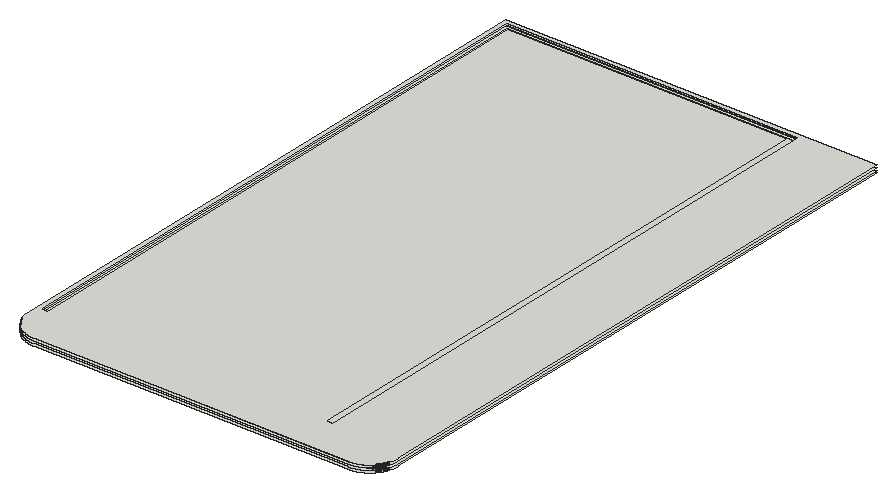
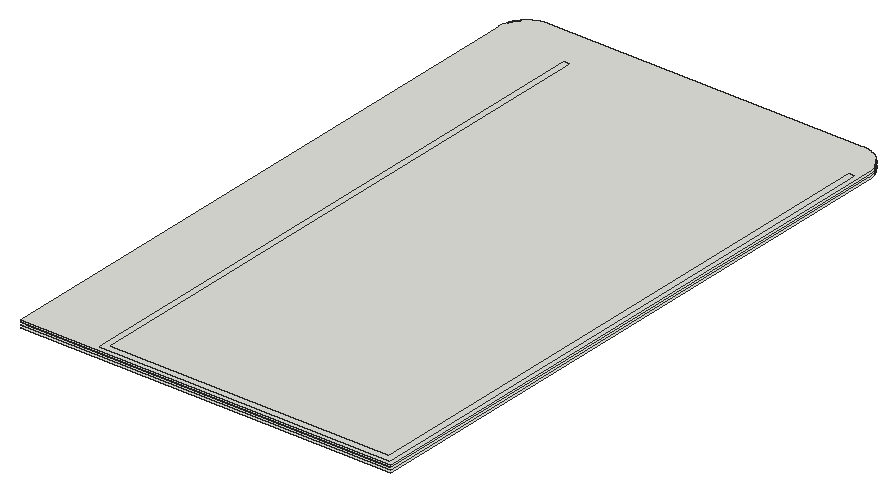
# SketchUp Ruby script. Lengths in inches.
U = 1.inch
M = Sketchup.active_model
def pt(a) = Geom::Point3d.new(a.map { |v| v * U })
def face(e, loops, mat)
  f = e.add_face(loops[0].map { |a| pt(a) })
  loops[1..].each { |l| e.add_face(l.map { |a| pt(a) }).erase! }
  f.material = f.back_material = mat if mat
  f
end
# faces: each face lists its corners as indices into pts; further lists are holes
def faces(e, pts, list, mat = nil) = list.each { |f| face(e, (f[0].is_a?(Array) ? f : [f]).map { |l| l.map { |i| pts[i] } }, mat) }
# xy, xz, yz: faces in a plane at the given z, y or x. An outline is a flat list of corners, or four numbers for a rectangle; further outlines are holes
def ring(l) = l.size == 4 ? [[l[0], l[1]], [l[2], l[1]], [l[2], l[3]], [l[0], l[3]]] : l.each_slice(2).to_a
def flat(e, list, mat, &to3) = list.each { |f| face(e, (f[0].is_a?(Array) ? f : [f]).map { |l| ring(l).map { |u, v| to3.(u, v) } }, mat) }
def xy(e, z, list, mat = nil) = flat(e, list, mat) { |x, y| [x, y, z] }
def xz(e, y, list, mat = nil) = flat(e, list, mat) { |x, z| [x, y, z] }
def yz(e, x, list, mat = nil) = flat(e, list, mat) { |y, z| [x, y, z] }
def lines(e, pts, list) = list.each { |a, b| e.add_line(pt(pts[a]), pt(pts[b])) }
# prism: a flat outline (further loops are holes) pulled along v
def prism(e, loops, v, mat = nil)
  f = face(e, loops, mat); d = Geom::Vector3d.new(v.map { |x| x * U })
  f.pushpull(f.normal.samedirection?(d) ? d.length : -d.length)
end
def box(e, o, s, mat = nil) = prism(e, [[o, [o[0] + s[0], o[1], o[2]], [o[0] + s[0], o[1] + s[1], o[2]], [o[0], o[1] + s[1], o[2]]]], [0, 0, s[2]], mat)
def at(x, y, z, deg = 0) = Geom::Transformation.translation(pt([x, y, z])) * Geom::Transformation.rotation(ORIGIN, Z_AXIS, deg.degrees)
def axes(o, x, y, z) = Geom::Transformation.new([*x, 0, *y, 0, *z, 0, *pt(o).to_a, 1])
def part(name) = M.definitions.add(name)
# library, detail: a bought-in or finely detailed component or shape, given as its bounding box
def library(name, o, s) = part(name).tap { |d| box(d.entities, o, s) }
def detail(e, o, s) = box(e.add_group.entities, o, s)
def put(e, d, t, mat = nil) = e.add_instance(d, t).tap { |i| i.material = mat if mat }
def group(e, t, mat = nil) = e.add_group.tap { |g| g.transformation = t; g.material = mat if mat }.entities
root = M.entities
xy(root,392.81,[[25.72,144,25.41,144.01,25.09,144.02,24.78,144.03,24.46,144.05,24.15,144.07,23.84,144.1,23.52,144.13,23.21,144.17,22.9,144.2,22.59,144.25,22.27,144.29,21.96,144.35,21.65,144.4,21.35,144.46,21.04,144.52,20.42,144.66,20.12,144.74,19.8125,144.82,19.51,144.9,18.61,145.17,18.31,145.27,18.01,145.375,17.72,145.48,17.42,145.59,16.26,146.07,15.97,146.2,15.6875,146.34,15.4,146.47,15.125,146.61,14.84,146.76,14.57,146.91,14.29,147.06,14.02,147.21,13.75,147.37,13.48,147.54,13.21,147.7,12.94,147.87,12.68,148.04,12.16,148.4,11.91,148.58,11.65,148.77,11.4,148.96,11.16,149.15,10.91,149.35,10.43,149.75,10.1875,149.95,9.95,150.16,9.49,150.59,9.26,150.81,8.82,151.25,8.6,151.48,8.39,151.71,8.17,151.94,7.96,152.17,7.56,152.65,7.36,152.9,7.16,153.14,6.59,153.89,6.41,154.15,6.23,154.4,6.05,154.67,5.71,155.19,5.54,155.46,5.06,156.27,4.91,156.55,4.76,156.82,4.48,157.38,4.34,157.67,4.21,157.95,4.08,158.24,3.95,158.52,3.83,158.8125,3.71,159.11,3.49,159.69,3.38,159.99,3.28,160.28,3.08,160.88,2.9,161.48,2.82,161.79,2.74,162.09,2.66,162.4,2.59,162.7,2.53,163.01,2.46,163.32,2.4,163.625,2.35,163.93,2.25,164.55,2.21,164.87,2.13,165.49,2.1,165.8,2.07,166.12,2.03,166.74,2.02,167.06,2,167.68,2,672,314.45,672,314.45,167.37,314.43,167.06,314.42,166.74,314.38,166.12,314.35,165.8,314.29,165.18,314.25,164.87,314.2,164.55,314.16,164.24,314.11,163.93,313.99,163.32,313.93,163.01,313.86,162.7,313.79,162.4,313.71,162.09,313.63,161.79,313.55,161.48,313.28,160.58,313.18,160.28,313.07,159.99,312.97,159.69,312.86,159.4,312.74,159.11,312.625,158.8125,312.5,158.52,312.375,158.24,312.25,157.95,312.11,157.67,311.97,157.38,311.83,157.1,311.6875,156.82,311.54,156.55,311.39,156.27,310.75,155.19,310.58,154.93,310.4,154.67,310.23,154.4,310.05,154.15,309.86,153.89,309.68,153.64,309.49,153.39,309.29,153.14,309.1,152.9,308.9,152.65,308.69,152.41,308.49,152.17,308.07,151.71,307.63,151.25,307.19,150.81,306.96,150.59,306.5,150.16,306.27,149.95,305.79,149.55,305.54,149.35,305.3,149.15,304.55,148.58,303.77,148.04,303.51,147.87,303.24,147.7,302.98,147.54,302.71,147.37,302.4375,147.21,302.16,147.06,301.89,146.91,301.33,146.61,301.05,146.47,300.77,146.34,300.48,146.2,300.19,146.07,299.91,145.95,299.62,145.83,299.32,145.71,299.03,145.59,298.74,145.48,298.14,145.27,297.85,145.17,297.55,145.08,297.24,144.99,296.94,144.9,296.64,144.82,296.33,144.74,296.03,144.66,295.72,144.59,295.42,144.52,294.8,144.4,294.49,144.35,294.18,144.29,293.87,144.25,293.56,144.2,293.24,144.17,292.93,144.13,292.62,144.1,292.3,144.07,291.68,144.03,291.36,144.02,291.05,144.01,290.73,144]])
xy(root,394.81,[[[25.72,144,290.73,144,291.05,144.01,291.36,144.02,291.68,144.03,292.3,144.07,292.62,144.1,292.93,144.13,293.24,144.17,293.56,144.2,293.87,144.25,294.18,144.29,294.49,144.35,294.8,144.4,295.42,144.52,295.72,144.59,296.03,144.66,296.33,144.74,296.64,144.82,296.94,144.9,297.24,144.99,297.55,145.08,297.85,145.17,298.14,145.27,298.74,145.48,299.03,145.59,299.32,145.71,299.62,145.83,299.91,145.95,300.19,146.07,300.48,146.2,300.77,146.34,301.05,146.47,301.33,146.61,301.89,146.91,302.16,147.06,302.4375,147.21,302.71,147.37,302.98,147.54,303.24,147.7,303.51,147.87,303.77,148.04,304.55,148.58,305.3,149.15,305.54,149.35,305.79,149.55,306.27,149.95,306.5,150.16,306.96,150.59,307.19,150.81,307.63,151.25,308.07,151.71,308.49,152.17,308.69,152.41,308.9,152.65,309.1,152.9,309.29,153.14,309.49,153.39,309.68,153.64,309.86,153.89,310.05,154.15,310.23,154.4,310.4,154.67,310.58,154.93,310.75,155.19,311.39,156.27,311.54,156.55,311.6875,156.82,311.83,157.1,311.97,157.38,312.11,157.67,312.25,157.95,312.375,158.24,312.5,158.52,312.625,158.8125,312.74,159.11,312.86,159.4,312.97,159.69,313.07,159.99,313.18,160.28,313.28,160.58,313.55,161.48,313.63,161.79,313.71,162.09,313.79,162.4,313.86,162.7,313.93,163.01,313.99,163.32,314.11,163.93,314.16,164.24,314.2,164.55,314.25,164.87,314.29,165.18,314.35,165.8,314.38,166.12,314.42,166.74,314.43,167.06,314.45,167.37,314.45,672,2,672,2,167.68,2.02,167.06,2.03,166.74,2.07,166.12,2.1,165.8,2.13,165.49,2.21,164.87,2.25,164.55,2.35,163.93,2.4,163.625,2.46,163.32,2.53,163.01,2.59,162.7,2.66,162.4,2.74,162.09,2.82,161.79,2.9,161.48,3.08,160.88,3.28,160.28,3.38,159.99,3.49,159.69,3.71,159.11,3.83,158.8125,3.95,158.52,4.08,158.24,4.21,157.95,4.34,157.67,4.48,157.38,4.76,156.82,4.91,156.55,5.06,156.27,5.54,155.46,5.71,155.19,6.05,154.67,6.23,154.4,6.41,154.15,6.59,153.89,7.16,153.14,7.36,152.9,7.56,152.65,7.96,152.17,8.17,151.94,8.39,151.71,8.6,151.48,8.82,151.25,9.26,150.81,9.49,150.59,9.95,150.16,10.1875,149.95,10.43,149.75,10.91,149.35,11.16,149.15,11.4,148.96,11.65,148.77,11.91,148.58,12.16,148.4,12.68,148.04,12.94,147.87,13.21,147.7,13.48,147.54,13.75,147.37,14.02,147.21,14.29,147.06,14.57,146.91,14.84,146.76,15.125,146.61,15.4,146.47,15.6875,146.34,15.97,146.2,16.26,146.07,17.42,145.59,17.72,145.48,18.01,145.375,18.31,145.27,18.61,145.17,19.51,144.9,19.8125,144.82,20.12,144.74,20.42,144.66,21.04,144.52,21.35,144.46,21.65,144.4,21.96,144.35,22.27,144.29,22.59,144.25,22.9,144.2,23.21,144.17,23.52,144.13,23.84,144.1,24.15,144.07,24.46,144.05,24.78,144.03,25.09,144.02,25.41,144.01],[25.75,146,24.88,146.03,24.59,146.05,24.31,146.07,24.02,146.09,23.44,146.15,23.16,146.1875,22.87,146.23,22.59,146.27,22.3,146.32,21.74,146.42,21.45,146.48,21.17,146.54,20.05,146.82,19.78,146.9,19.22,147.08,18.68,147.26,18.14,147.46,17.87,147.57,17.6,147.67,17.34,147.79,17.07,147.9,16.55,148.14,15.77,148.53,15.52,148.67,15.27,148.8,15.02,148.95,14.77,149.09,14.52,149.24,14.28,149.39,14.03,149.55,13.55,149.87,13.32,150.03,13.08,150.2,12.85,150.37,12.62,150.55,12.39,150.72,12.17,150.9,11.94,151.09,11.72,151.27,11.51,151.46,11.29,151.65,11.08,151.84,10.45,152.44,9.85,153.07,9.47,153.49,9.09,153.93,8.91,154.15,8.55,154.61,8.04,155.3,7.71,155.78,7.55,156.02,7.25,156.5,6.95,157,6.67,157.5,6.53,157.76,6.4,158.01,6.27,158.27,6.15,158.53,6.02,158.79,5.9,159.05,5.79,159.32,5.68,159.58,5.46,160.12,5.26,160.66,5.08,161.2,4.99,161.48,4.91,161.75,4.75,162.31,4.68,162.58,4.54,163.14,4.48,163.43,4.42,163.71,4.32,164.27,4.27,164.56,4.23,164.84,4.1875,165.13,4.15,165.41,4.09,165.99,4.07,166.27,4.03,166.85,4.02,167.14,4.01,167.42,4,167.71,4,670,312.45,670,312.45,167.42,312.4375,167.14,312.42,166.85,312.41,166.56,312.39,166.27,312.36,165.99,312.3,165.41,312.26,165.13,312.23,164.84,312.18,164.56,312.14,164.27,312.08,163.99,312.03,163.71,311.97,163.43,311.91,163.14,311.84,162.86,311.78,162.58,311.7,162.31,311.55,161.75,311.46,161.48,311.375,161.2,311.28,160.93,311.19,160.66,310.89,159.85,310.78,159.58,310.66,159.32,310.55,159.05,310.31,158.53,310.05,158.01,309.92,157.76,309.78,157.5,309.36,156.75,309.21,156.5,309.05,156.26,308.9,156.02,308.58,155.54,308.41,155.3,308.25,155.07,308.07,154.84,307.9,154.61,307.54,154.15,307.36,153.93,307.17,153.71,306.99,153.49,306.79,153.28,306.6,153.07,306,152.44,305.8,152.24,305.59,152.04,305.375,151.84,305.16,151.65,304.95,151.46,304.73,151.27,304.51,151.09,304.29,150.9,304.0625,150.72,303.83,150.55,303.6,150.37,303.14,150.03,302.18,149.39,301.93,149.24,301.6875,149.09,301.4375,148.95,301.1875,148.8,300.93,148.67,300.68,148.53,300.42,148.4,300.17,148.27,299.91,148.14,299.64,148.02,299.38,147.9,299.12,147.79,298.85,147.67,298.58,147.57,298.32,147.46,298.05,147.36,297.77,147.26,297.23,147.08,296.95,146.99,296.68,146.9,296.4,146.82,295.84,146.68,295.5625,146.61,295.28,146.54,294.72,146.42,294.43,146.37,293.87,146.27,293.58,146.23,293.3,146.1875,293.01,146.15,292.72,146.12,292.44,146.09,291.57,146.03,291.28,146.02,291,146.01,290.71,146]]])
xy(root,396.81,[[[25.72,144,25.41,144.01,25.09,144.02,24.78,144.03,24.46,144.05,24.15,144.07,23.84,144.1,23.52,144.13,23.21,144.17,22.9,144.2,22.59,144.25,22.27,144.29,21.96,144.35,21.65,144.4,21.35,144.46,21.04,144.52,20.42,144.66,20.12,144.74,19.8125,144.82,19.51,144.9,18.61,145.17,18.31,145.27,18.01,145.375,17.72,145.48,17.42,145.59,16.26,146.07,15.97,146.2,15.6875,146.34,15.4,146.47,15.125,146.61,14.84,146.76,14.57,146.91,14.29,147.06,14.02,147.21,13.75,147.37,13.48,147.54,13.21,147.7,12.94,147.87,12.68,148.04,12.16,148.4,11.91,148.58,11.65,148.77,11.4,148.96,11.16,149.15,10.91,149.35,10.43,149.75,10.1875,149.95,9.95,150.16,9.49,150.59,9.26,150.81,8.82,151.25,8.6,151.48,8.39,151.71,8.17,151.94,7.96,152.17,7.56,152.65,7.36,152.9,7.16,153.14,6.59,153.89,6.41,154.15,6.23,154.4,6.05,154.67,5.71,155.19,5.54,155.46,5.06,156.27,4.91,156.55,4.76,156.82,4.48,157.38,4.34,157.67,4.21,157.95,4.08,158.24,3.95,158.52,3.83,158.8125,3.71,159.11,3.49,159.69,3.38,159.99,3.28,160.28,3.08,160.88,2.9,161.48,2.82,161.79,2.74,162.09,2.66,162.4,2.59,162.7,2.53,163.01,2.46,163.32,2.4,163.625,2.35,163.93,2.25,164.55,2.21,164.87,2.13,165.49,2.1,165.8,2.07,166.12,2.03,166.74,2.02,167.06,2,167.68,2,672,314.45,672,314.45,167.37,314.43,167.06,314.42,166.74,314.38,166.12,314.35,165.8,314.29,165.18,314.25,164.87,314.2,164.55,314.16,164.24,314.11,163.93,313.99,163.32,313.93,163.01,313.86,162.7,313.79,162.4,313.71,162.09,313.63,161.79,313.55,161.48,313.28,160.58,313.18,160.28,313.07,159.99,312.97,159.69,312.86,159.4,312.74,159.11,312.625,158.8125,312.5,158.52,312.375,158.24,312.25,157.95,312.11,157.67,311.97,157.38,311.83,157.1,311.6875,156.82,311.54,156.55,311.39,156.27,310.75,155.19,310.58,154.93,310.4,154.67,310.23,154.4,310.05,154.15,309.86,153.89,309.68,153.64,309.49,153.39,309.29,153.14,309.1,152.9,308.9,152.65,308.69,152.41,308.49,152.17,308.07,151.71,307.63,151.25,307.19,150.81,306.96,150.59,306.5,150.16,306.27,149.95,305.79,149.55,305.54,149.35,305.3,149.15,304.55,148.58,303.77,148.04,303.51,147.87,303.24,147.7,302.98,147.54,302.71,147.37,302.4375,147.21,302.16,147.06,301.89,146.91,301.33,146.61,301.05,146.47,300.77,146.34,300.48,146.2,300.19,146.07,299.91,145.95,299.62,145.83,299.32,145.71,299.03,145.59,298.74,145.48,298.14,145.27,297.85,145.17,297.55,145.08,297.24,144.99,296.94,144.9,296.64,144.82,296.33,144.74,296.03,144.66,295.72,144.59,295.42,144.52,294.8,144.4,294.49,144.35,294.18,144.29,293.87,144.25,293.56,144.2,293.24,144.17,292.93,144.13,292.62,144.1,292.3,144.07,291.68,144.03,291.36,144.02,291.05,144.01,290.73,144],[25.75,146,290.71,146,291,146.01,291.28,146.02,291.57,146.03,292.44,146.09,292.72,146.12,293.01,146.15,293.3,146.1875,293.58,146.23,293.87,146.27,294.43,146.37,294.72,146.42,295.28,146.54,295.5625,146.61,295.84,146.68,296.4,146.82,296.68,146.9,296.95,146.99,297.23,147.08,297.77,147.26,298.05,147.36,298.32,147.46,298.58,147.57,298.85,147.67,299.12,147.79,299.38,147.9,299.64,148.02,299.91,148.14,300.17,148.27,300.42,148.4,300.68,148.53,300.93,148.67,301.1875,148.8,301.4375,148.95,301.6875,149.09,301.93,149.24,302.18,149.39,303.14,150.03,303.6,150.37,303.83,150.55,304.0625,150.72,304.29,150.9,304.51,151.09,304.73,151.27,304.95,151.46,305.16,151.65,305.375,151.84,305.59,152.04,305.8,152.24,306,152.44,306.6,153.07,306.79,153.28,306.99,153.49,307.17,153.71,307.36,153.93,307.54,154.15,307.9,154.61,308.07,154.84,308.25,155.07,308.41,155.3,308.58,155.54,308.9,156.02,309.05,156.26,309.21,156.5,309.36,156.75,309.78,157.5,309.92,157.76,310.05,158.01,310.31,158.53,310.55,159.05,310.66,159.32,310.78,159.58,310.89,159.85,311.19,160.66,311.28,160.93,311.375,161.2,311.46,161.48,311.55,161.75,311.7,162.31,311.78,162.58,311.84,162.86,311.91,163.14,311.97,163.43,312.03,163.71,312.08,163.99,312.14,164.27,312.18,164.56,312.23,164.84,312.26,165.13,312.3,165.41,312.36,165.99,312.39,166.27,312.41,166.56,312.42,166.85,312.4375,167.14,312.45,167.42,312.45,670,4,670,4,167.71,4.01,167.42,4.02,167.14,4.03,166.85,4.07,166.27,4.09,165.99,4.15,165.41,4.1875,165.13,4.23,164.84,4.27,164.56,4.32,164.27,4.42,163.71,4.48,163.43,4.54,163.14,4.68,162.58,4.75,162.31,4.91,161.75,4.99,161.48,5.08,161.2,5.26,160.66,5.46,160.12,5.68,159.58,5.79,159.32,5.9,159.05,6.02,158.79,6.15,158.53,6.27,158.27,6.4,158.01,6.53,157.76,6.67,157.5,6.95,157,7.25,156.5,7.55,156.02,7.71,155.78,8.04,155.3,8.55,154.61,8.91,154.15,9.09,153.93,9.47,153.49,9.85,153.07,10.45,152.44,11.08,151.84,11.29,151.65,11.51,151.46,11.72,151.27,11.94,151.09,12.17,150.9,12.39,150.72,12.62,150.55,12.85,150.37,13.08,150.2,13.32,150.03,13.55,149.87,14.03,149.55,14.28,149.39,14.52,149.24,14.77,149.09,15.02,148.95,15.27,148.8,15.52,148.67,15.77,148.53,16.55,148.14,17.07,147.9,17.34,147.79,17.6,147.67,17.87,147.57,18.14,147.46,18.68,147.26,19.22,147.08,19.78,146.9,20.05,146.82,21.17,146.54,21.45,146.48,21.74,146.42,22.3,146.32,22.59,146.27,22.87,146.23,23.16,146.1875,23.44,146.15,24.02,146.09,24.31,146.07,24.59,146.05,24.88,146.03]]])
xy(root,398.81,[[[25.72,144,290.73,144,291.05,144.01,291.36,144.02,291.68,144.03,292.3,144.07,292.62,144.1,292.93,144.13,293.24,144.17,293.56,144.2,293.87,144.25,294.18,144.29,294.49,144.35,294.8,144.4,295.42,144.52,295.72,144.59,296.03,144.66,296.33,144.74,296.64,144.82,296.94,144.9,297.24,144.99,297.55,145.08,297.85,145.17,298.14,145.27,298.74,145.48,299.03,145.59,299.32,145.71,299.62,145.83,299.91,145.95,300.19,146.07,300.48,146.2,300.77,146.34,301.05,146.47,301.33,146.61,301.89,146.91,302.16,147.06,302.4375,147.21,302.71,147.37,302.98,147.54,303.24,147.7,303.51,147.87,303.77,148.04,304.55,148.58,305.3,149.15,305.54,149.35,305.79,149.55,306.27,149.95,306.5,150.16,306.96,150.59,307.19,150.81,307.63,151.25,308.07,151.71,308.49,152.17,308.69,152.41,308.9,152.65,309.1,152.9,309.29,153.14,309.49,153.39,309.68,153.64,309.86,153.89,310.05,154.15,310.23,154.4,310.4,154.67,310.58,154.93,310.75,155.19,311.39,156.27,311.54,156.55,311.6875,156.82,311.83,157.1,311.97,157.38,312.11,157.67,312.25,157.95,312.375,158.24,312.5,158.52,312.625,158.8125,312.74,159.11,312.86,159.4,312.97,159.69,313.07,159.99,313.18,160.28,313.28,160.58,313.55,161.48,313.63,161.79,313.71,162.09,313.79,162.4,313.86,162.7,313.93,163.01,313.99,163.32,314.11,163.93,314.16,164.24,314.2,164.55,314.25,164.87,314.29,165.18,314.35,165.8,314.38,166.12,314.42,166.74,314.43,167.06,314.45,167.37,314.45,672,2,672,2,167.68,2.02,167.06,2.03,166.74,2.07,166.12,2.1,165.8,2.13,165.49,2.21,164.87,2.25,164.55,2.35,163.93,2.4,163.625,2.46,163.32,2.53,163.01,2.59,162.7,2.66,162.4,2.74,162.09,2.82,161.79,2.9,161.48,3.08,160.88,3.28,160.28,3.38,159.99,3.49,159.69,3.71,159.11,3.83,158.8125,3.95,158.52,4.08,158.24,4.21,157.95,4.34,157.67,4.48,157.38,4.76,156.82,4.91,156.55,5.06,156.27,5.54,155.46,5.71,155.19,6.05,154.67,6.23,154.4,6.41,154.15,6.59,153.89,7.16,153.14,7.36,152.9,7.56,152.65,7.96,152.17,8.17,151.94,8.39,151.71,8.6,151.48,8.82,151.25,9.26,150.81,9.49,150.59,9.95,150.16,10.1875,149.95,10.43,149.75,10.91,149.35,11.16,149.15,11.4,148.96,11.65,148.77,11.91,148.58,12.16,148.4,12.68,148.04,12.94,147.87,13.21,147.7,13.48,147.54,13.75,147.37,14.02,147.21,14.29,147.06,14.57,146.91,14.84,146.76,15.125,146.61,15.4,146.47,15.6875,146.34,15.97,146.2,16.26,146.07,17.42,145.59,17.72,145.48,18.01,145.375,18.31,145.27,18.61,145.17,19.51,144.9,19.8125,144.82,20.12,144.74,20.42,144.66,21.04,144.52,21.35,144.46,21.65,144.4,21.96,144.35,22.27,144.29,22.59,144.25,22.9,144.2,23.21,144.17,23.52,144.13,23.84,144.1,24.15,144.07,24.46,144.05,24.78,144.03,25.09,144.02,25.41,144.01],[5,177.03,5,669,251.45,669,251.45,177.03,245.45,177.03,245.45,663,11,663,11,177.03]]])
p = [[7.96,152.17,392.81],[8.17,151.94,392.81],[8.17,151.94,394.81],[7.96,152.17,394.81],[308.28,151.94,392.81],[308.49,152.17,392.81],
  [308.49,152.17,394.81],[308.28,151.94,394.81],[7.76,152.41,392.81],[7.76,152.41,394.81],[308.69,152.41,392.81],[308.69,152.41,394.81],
  [7.56,152.65,392.81],[7.56,152.65,394.81],[308.9,152.65,392.81],[308.9,152.65,394.81],[7.36,152.9,392.81],[7.36,152.9,394.81],
  [309.1,152.9,392.81],[309.1,152.9,394.81],[7.16,153.14,392.81],[7.16,153.14,394.81],[309.29,153.14,392.81],[309.29,153.14,394.81],
  [6.97,153.39,392.81],[6.97,153.39,394.81],[309.49,153.39,392.81],[309.49,153.39,394.81],[6.78,153.64,392.81],[6.78,153.64,394.81],
  [309.68,153.64,392.81],[309.68,153.64,394.81],[6.59,153.89,392.81],[6.59,153.89,394.81],[309.86,153.89,392.81],[309.86,153.89,394.81],
  [6.41,154.15,392.81],[6.41,154.15,394.81],[310.05,154.15,392.81],[310.05,154.15,394.81],[6.23,154.4,392.81],[6.23,154.4,394.81],
  [310.23,154.4,392.81],[310.23,154.4,394.81],[6.05,154.67,392.81],[6.05,154.67,394.81],[310.4,154.67,392.81],[310.4,154.67,394.81],
  [5.88,154.93,392.81],[5.88,154.93,394.81],[310.58,154.93,392.81],[310.58,154.93,394.81],[5.71,155.19,392.81],[5.71,155.19,394.81],
  [310.75,155.19,392.81],[310.75,155.19,394.81],[5.54,155.46,392.81],[5.54,155.46,394.81],[310.91,155.46,392.81],[310.91,155.46,394.81],
  [5.38,155.73,392.81],[5.38,155.73,394.81],[311.07,155.73,392.81],[311.07,155.73,394.81],[5.22,156,392.81],[5.22,156,394.81],
  [311.23,156,392.81],[311.23,156,394.81],[5.06,156.27,392.81],[5.06,156.27,394.81],[311.39,156.27,392.81],[311.39,156.27,394.81],
  [4.91,156.55,392.81],[4.91,156.55,394.81],[311.54,156.55,392.81],[311.54,156.55,394.81],[4.76,156.82,392.81],[4.76,156.82,394.81],
  [311.6875,156.82,392.81],[311.6875,156.82,394.81],[4.62,157.1,392.81],[4.62,157.1,394.81],[311.83,157.1,392.81],[311.83,157.1,394.81],
  [4.48,157.38,392.81],[4.48,157.38,394.81],[311.97,157.38,392.81],[311.97,157.38,394.81],[4.34,157.67,392.81],[4.34,157.67,394.81],
  [312.11,157.67,392.81],[312.11,157.67,394.81],[4.21,157.95,392.81],[4.21,157.95,394.81],[312.25,157.95,392.81],[312.25,157.95,394.81],
  [4.08,158.24,392.81],[4.08,158.24,394.81],[312.375,158.24,392.81],[312.375,158.24,394.81],[3.95,158.52,392.81],[3.95,158.52,394.81],
  [312.5,158.52,392.81],[312.5,158.52,394.81],[3.83,158.8125,392.81],[3.83,158.8125,394.81],[312.625,158.8125,392.81],[312.625,158.8125,394.81],
  [3.71,159.11,392.81],[3.71,159.11,394.81],[312.74,159.11,392.81],[312.74,159.11,394.81],[3.6,159.4,392.81],[3.6,159.4,394.81],
  [312.86,159.4,392.81],[312.86,159.4,394.81],[3.49,159.69,392.81],[3.49,159.69,394.81],[312.97,159.69,392.81],[312.97,159.69,394.81],
  [305.375,151.84,394.81],[305.59,152.04,394.81],[305.59,152.04,396.81],[305.375,151.84,396.81],[10.66,152.24,394.81],[10.87,152.04,394.81],
  [10.87,152.04,396.81],[10.66,152.24,396.81],[305.8,152.24,394.81],[305.8,152.24,396.81],[10.45,152.44,394.81],[10.45,152.44,396.81],
  [306,152.44,394.81],[306,152.44,396.81],[10.25,152.65,394.81],[10.25,152.65,396.81],[306.2,152.65,394.81],[306.2,152.65,396.81],
  [10.05,152.86,394.81],[10.05,152.86,396.81],[306.4,152.86,394.81],[306.4,152.86,396.81],[9.85,153.07,394.81],[9.85,153.07,396.81],
  [306.6,153.07,394.81],[306.6,153.07,396.81],[9.66,153.28,394.81],[9.66,153.28,396.81],[306.79,153.28,394.81],[306.79,153.28,396.81],
  [9.47,153.49,394.81],[9.47,153.49,396.81],[306.99,153.49,394.81],[306.99,153.49,396.81],[9.28,153.71,394.81],[9.28,153.71,396.81],
  [307.17,153.71,394.81],[307.17,153.71,396.81],[9.09,153.93,394.81],[9.09,153.93,396.81],[307.36,153.93,394.81],[307.36,153.93,396.81],
  [8.91,154.15,394.81],[8.91,154.15,396.81],[307.54,154.15,394.81],[307.54,154.15,396.81],[8.73,154.38,394.81],[8.73,154.38,396.81],
  [307.72,154.38,394.81],[307.72,154.38,396.81],[8.55,154.61,394.81],[8.55,154.61,396.81],[307.9,154.61,394.81],[307.9,154.61,396.81],
  [8.38,154.84,394.81],[8.38,154.84,396.81],[308.07,154.84,394.81],[308.07,154.84,396.81],[8.21,155.07,394.81],[8.21,155.07,396.81],
  [308.25,155.07,394.81],[308.25,155.07,396.81],[8.04,155.3,394.81],[8.04,155.3,396.81],[308.41,155.3,394.81],[308.41,155.3,396.81],
  [7.875,155.54,394.81],[7.875,155.54,396.81],[308.58,155.54,394.81],[308.58,155.54,396.81],[7.71,155.78,394.81],[7.71,155.78,396.81],
  [308.74,155.78,394.81],[308.74,155.78,396.81],[7.55,156.02,394.81],[7.55,156.02,396.81],[308.9,156.02,394.81],[308.9,156.02,396.81],
  [7.4,156.26,394.81],[7.4,156.26,396.81],[309.05,156.26,394.81],[309.05,156.26,396.81],[7.25,156.5,394.81],[7.25,156.5,396.81],
  [309.21,156.5,394.81],[309.21,156.5,396.81],[7.1,156.75,394.81],[7.1,156.75,396.81],[309.36,156.75,394.81],[309.36,156.75,396.81],
  [6.95,157,394.81],[6.95,157,396.81],[309.5,157,394.81],[309.5,157,396.81],[6.81,157.25,394.81],[6.81,157.25,396.81],
  [309.64,157.25,394.81],[309.64,157.25,396.81],[6.67,157.5,394.81],[6.67,157.5,396.81],[309.78,157.5,394.81],[309.78,157.5,396.81],
  [6.53,157.76,394.81],[6.53,157.76,396.81],[309.92,157.76,394.81],[309.92,157.76,396.81],[6.4,158.01,394.81],[6.4,158.01,396.81],
  [310.05,158.01,394.81],[310.05,158.01,396.81],[6.27,158.27,394.81],[6.27,158.27,396.81],[310.18,158.27,394.81],[310.18,158.27,396.81],
  [6.15,158.53,394.81],[6.15,158.53,396.81],[310.31,158.53,394.81],[310.31,158.53,396.81],[6.02,158.79,394.81],[6.02,158.79,396.81],
  [310.43,158.79,394.81],[310.43,158.79,396.81],[5.9,159.05,394.81],[5.9,159.05,396.81],[310.55,159.05,394.81],[310.55,159.05,396.81],
  [5.79,159.32,394.81],[5.79,159.32,396.81],[310.66,159.32,394.81],[310.66,159.32,396.81],[5.68,159.58,394.81],[5.68,159.58,396.81],
  [310.78,159.58,394.81],[310.78,159.58,396.81],[5.57,159.85,394.81],[5.57,159.85,396.81],[310.89,159.85,394.81],[310.89,159.85,396.81],
  [7.96,152.17,396.81],[8.17,151.94,396.81],[8.17,151.94,398.81],[7.96,152.17,398.81],[308.28,151.94,396.81],[308.49,152.17,396.81],
  [308.49,152.17,398.81],[308.28,151.94,398.81],[7.76,152.41,396.81],[7.76,152.41,398.81],[308.69,152.41,396.81],[308.69,152.41,398.81],
  [7.56,152.65,396.81],[7.56,152.65,398.81],[308.9,152.65,396.81],[308.9,152.65,398.81],[7.36,152.9,396.81],[7.36,152.9,398.81],
  [309.1,152.9,396.81],[309.1,152.9,398.81],[7.16,153.14,396.81],[7.16,153.14,398.81],[309.29,153.14,396.81],[309.29,153.14,398.81],
  [6.97,153.39,396.81],[6.97,153.39,398.81],[309.49,153.39,396.81],[309.49,153.39,398.81],[6.78,153.64,396.81],[6.78,153.64,398.81],
  [309.68,153.64,396.81],[309.68,153.64,398.81],[6.59,153.89,396.81],[6.59,153.89,398.81],[309.86,153.89,396.81],[309.86,153.89,398.81],
  [6.41,154.15,396.81],[6.41,154.15,398.81],[310.05,154.15,396.81],[310.05,154.15,398.81],[6.23,154.4,396.81],[6.23,154.4,398.81],
  [310.23,154.4,396.81],[310.23,154.4,398.81],[6.05,154.67,396.81],[6.05,154.67,398.81],[310.4,154.67,396.81],[310.4,154.67,398.81],
  [5.88,154.93,396.81],[5.88,154.93,398.81],[310.58,154.93,396.81],[310.58,154.93,398.81],[5.71,155.19,396.81],[5.71,155.19,398.81],
  [310.75,155.19,396.81],[310.75,155.19,398.81],[5.54,155.46,396.81],[5.54,155.46,398.81],[310.91,155.46,396.81],[310.91,155.46,398.81],
  [5.38,155.73,396.81],[5.38,155.73,398.81],[311.07,155.73,396.81],[311.07,155.73,398.81],[5.22,156,396.81],[5.22,156,398.81],
  [311.23,156,396.81],[311.23,156,398.81],[5.06,156.27,396.81],[5.06,156.27,398.81],[311.39,156.27,396.81],[311.39,156.27,398.81],
  [4.91,156.55,396.81],[4.91,156.55,398.81],[311.54,156.55,396.81],[311.54,156.55,398.81],[4.76,156.82,396.81],[4.76,156.82,398.81],
  [311.6875,156.82,396.81],[311.6875,156.82,398.81],[4.62,157.1,396.81],[4.62,157.1,398.81],[311.83,157.1,396.81],[311.83,157.1,398.81],
  [4.48,157.38,396.81],[4.48,157.38,398.81],[311.97,157.38,396.81],[311.97,157.38,398.81],[4.34,157.67,396.81],[4.34,157.67,398.81],
  [312.11,157.67,396.81],[312.11,157.67,398.81],[4.21,157.95,396.81],[4.21,157.95,398.81],[312.25,157.95,396.81],[312.25,157.95,398.81],
  [4.08,158.24,396.81],[4.08,158.24,398.81],[312.375,158.24,396.81],[312.375,158.24,398.81],[3.95,158.52,396.81],[3.95,158.52,398.81],
  [312.5,158.52,396.81],[312.5,158.52,398.81],[3.83,158.8125,396.81],[3.83,158.8125,398.81],[312.625,158.8125,396.81],[312.625,158.8125,398.81],
  [3.71,159.11,396.81],[3.71,159.11,398.81],[312.74,159.11,396.81],[312.74,159.11,398.81],[3.6,159.4,396.81],[3.6,159.4,398.81],
  [312.86,159.4,396.81],[312.86,159.4,398.81],[3.49,159.69,396.81],[3.49,159.69,398.81],[312.97,159.69,396.81],[312.97,159.69,398.81]]
faces(root,p,[[0,1,2,3],[4,5,6,7],[8,0,3,9],[5,10,11,6],[12,8,9,13],[10,14,15,11],[16,12,13,17],[14,18,19,15],
  [20,16,17,21],[18,22,23,19],[24,20,21,25],[22,26,27,23],[28,24,25,29],[26,30,31,27],[32,28,29,33],[30,34,35,31],
  [36,32,33,37],[34,38,39,35],[40,36,37,41],[38,42,43,39],[44,40,41,45],[42,46,47,43],[48,44,45,49],[46,50,51,47],
  [52,48,49,53],[50,54,55,51],[56,52,53,57],[54,58,59,55],[60,56,57,61],[58,62,63,59],[64,60,61,65],[62,66,67,63],
  [68,64,65,69],[66,70,71,67],[72,68,69,73],[70,74,75,71],[76,72,73,77],[74,78,79,75],[80,76,77,81],[78,82,83,79],
  [84,80,81,85],[82,86,87,83],[88,84,85,89],[86,90,91,87],[92,88,89,93],[90,94,95,91],[96,92,93,97],[94,98,99,95],
  [100,96,97,101],[98,102,103,99],[104,100,101,105],[102,106,107,103],[108,104,105,109],[106,110,111,107],[112,108,109,113],[110,114,115,111],
  [116,112,113,117],[114,118,119,115],[120,121,122,123],[124,125,126,127],[121,128,129,122],[130,124,127,131],[128,132,133,129],[134,130,131,135],
  [132,136,137,133],[138,134,135,139],[136,140,141,137],[142,138,139,143],[140,144,145,141],[146,142,143,147],[144,148,149,145],[150,146,147,151],
  [148,152,153,149],[154,150,151,155],[152,156,157,153],[158,154,155,159],[156,160,161,157],[162,158,159,163],[160,164,165,161],[166,162,163,167],
  [164,168,169,165],[170,166,167,171],[168,172,173,169],[174,170,171,175],[172,176,177,173],[178,174,175,179],[176,180,181,177],[182,178,179,183],
  [180,184,185,181],[186,182,183,187],[184,188,189,185],[190,186,187,191],[188,192,193,189],[194,190,191,195],[192,196,197,193],[198,194,195,199],
  [196,200,201,197],[202,198,199,203],[200,204,205,201],[206,202,203,207],[204,208,209,205],[210,206,207,211],[208,212,213,209],[214,210,211,215],
  [212,216,217,213],[218,214,215,219],[216,220,221,217],[222,218,219,223],[220,224,225,221],[226,222,223,227],[224,228,229,225],[230,226,227,231],
  [228,232,233,229],[234,230,231,235],[232,236,237,233],[238,234,235,239],[236,240,241,237],[242,238,239,243],[240,244,245,241],[246,242,243,247],
  [244,248,249,245],[250,246,247,251],[248,252,253,249],[254,250,251,255],[252,256,257,253],[258,259,260,261],[262,263,264,265],[266,258,261,267],
  [263,268,269,264],[270,266,267,271],[268,272,273,269],[274,270,271,275],[272,276,277,273],[278,274,275,279],[276,280,281,277],[282,278,279,283],
  [280,284,285,281],[286,282,283,287],[284,288,289,285],[290,286,287,291],[288,292,293,289],[294,290,291,295],[292,296,297,293],[298,294,295,299],
  [296,300,301,297],[302,298,299,303],[300,304,305,301],[306,302,303,307],[304,308,309,305],[310,306,307,311],[308,312,313,309],[314,310,311,315],
  [312,316,317,313],[318,314,315,319],[316,320,321,317],[322,318,319,323],[320,324,325,321],[326,322,323,327],[324,328,329,325],[330,326,327,331],
  [328,332,333,329],[334,330,331,335],[332,336,337,333],[338,334,335,339],[336,340,341,337],[342,338,339,343],[340,344,345,341],[346,342,343,347],
  [344,348,349,345],[350,346,347,351],[348,352,353,349],[354,350,351,355],[352,356,357,353],[358,354,355,359],[356,360,361,357],[362,358,359,363],
  [360,364,365,361],[366,362,363,367],[364,368,369,365],[370,366,367,371],[368,372,373,369],[374,370,371,375],[372,376,377,373]])
